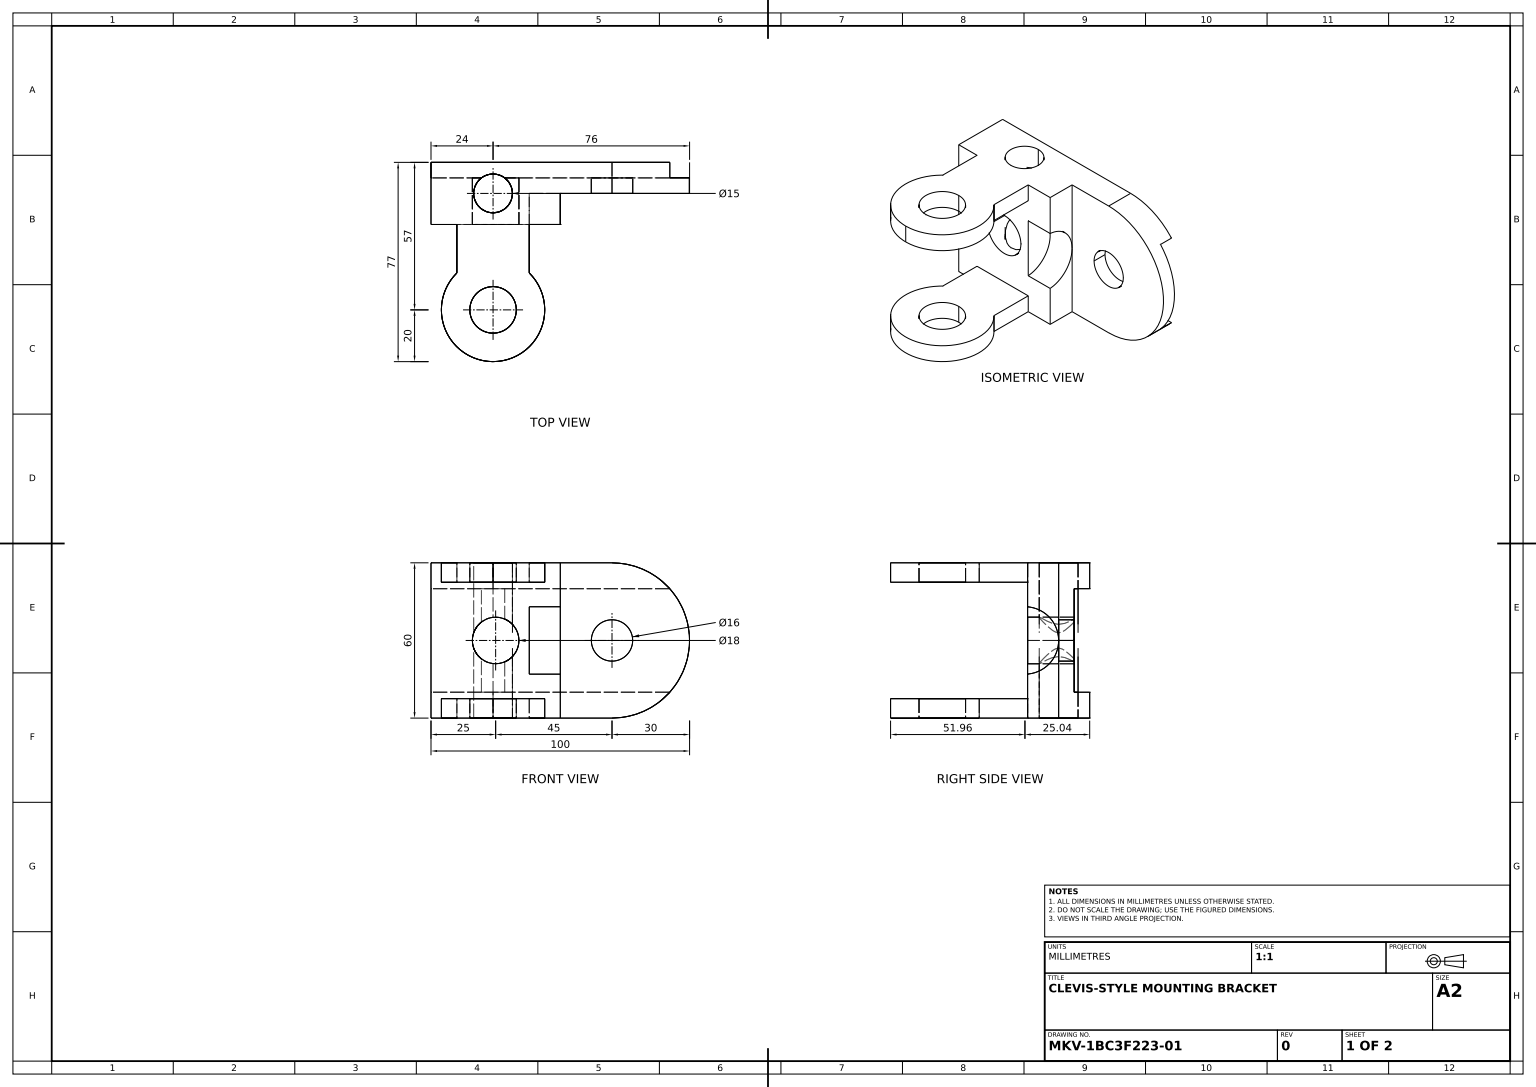
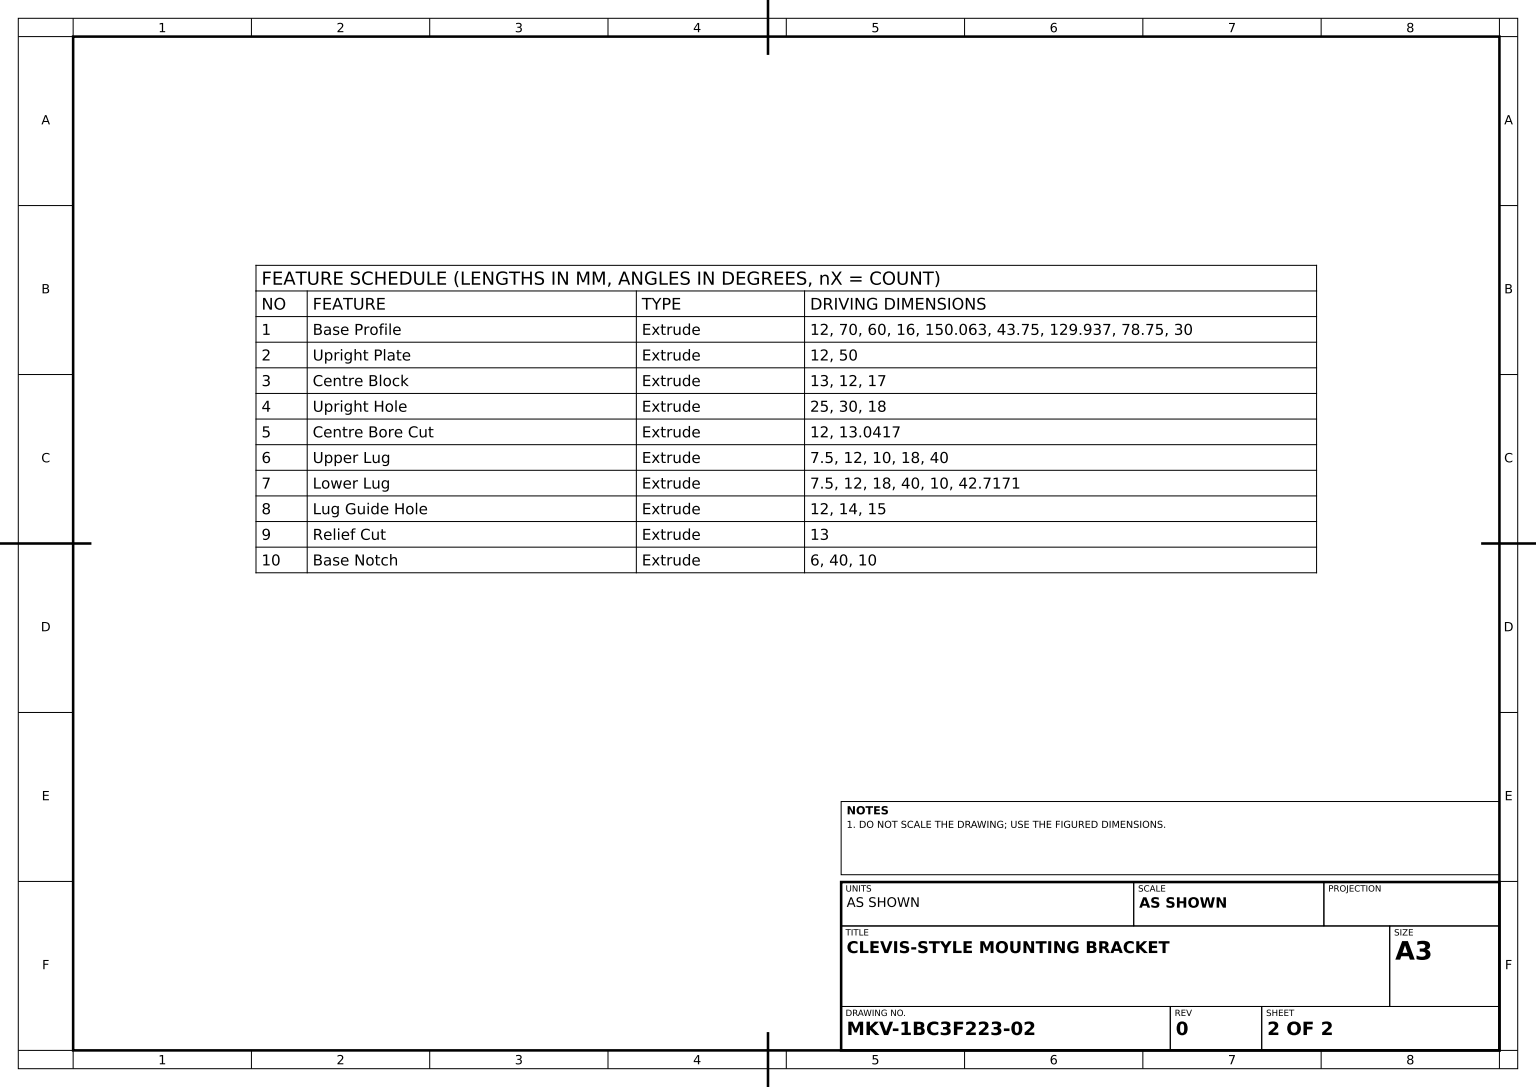
ISO-10303-21;
HEADER;
FILE_DESCRIPTION((''),'2;1');
FILE_NAME('','',(''),(''),'','','');
FILE_SCHEMA(('AUTOMOTIVE_DESIGN'));
ENDSEC;
DATA;
#1=APPLICATION_CONTEXT('');
#2=PRODUCT_CONTEXT('',#1,'mechanical');
#3=PRODUCT('','','',(#2));
#4=PRODUCT_DEFINITION_FORMATION('','',#3);
#5=PRODUCT_DEFINITION_CONTEXT('',#1,'design');
#6=PRODUCT_DEFINITION('','',#4,#5);
#7=PRODUCT_DEFINITION_SHAPE('','',#6);
#8=(LENGTH_UNIT()NAMED_UNIT(*)SI_UNIT(.MILLI.,.METRE.));
#9=(NAMED_UNIT(*)PLANE_ANGLE_UNIT()SI_UNIT($,.RADIAN.));
#10=(NAMED_UNIT(*)SI_UNIT($,.STERADIAN.)SOLID_ANGLE_UNIT());
#11=UNCERTAINTY_MEASURE_WITH_UNIT(LENGTH_MEASURE(1.E-05),#8,'distance_accuracy_value','');
#12=(GEOMETRIC_REPRESENTATION_CONTEXT(3)GLOBAL_UNCERTAINTY_ASSIGNED_CONTEXT((#11))GLOBAL_UNIT_ASSIGNED_CONTEXT((#8,#9,#10))REPRESENTATION_CONTEXT('',''));
#13=CARTESIAN_POINT('',(78.,30.,6.));
#14=VERTEX_POINT('',#13);
#15=CARTESIAN_POINT('',(78.,30.,0.));
#16=VERTEX_POINT('',#15);
#17=DIRECTION('',(0.,0.,-1.));
#18=VECTOR('',#17,1000.);
#19=LINE('',#13,#18);
#20=EDGE_CURVE('',#14,#16,#19,.T.);
#21=ORIENTED_EDGE('',*,*,#20,.F.);
#22=CARTESIAN_POINT('',(62.,30.,6.));
#23=VERTEX_POINT('',#22);
#24=CARTESIAN_POINT('',(70.,30.,6.));
#25=DIRECTION('',(0.,0.,1.));
#26=DIRECTION('',(1.,0.,0.));
#27=AXIS2_PLACEMENT_3D('',#24,#25,#26);
#28=CIRCLE('',#27,8.);
#29=EDGE_CURVE('',#14,#23,#28,.T.);
#30=ORIENTED_EDGE('',*,*,#29,.T.);
#31=CARTESIAN_POINT('',(62.,30.,0.));
#32=VERTEX_POINT('',#31);
#33=LINE('',#22,#18);
#34=EDGE_CURVE('',#23,#32,#33,.T.);
#35=ORIENTED_EDGE('',*,*,#34,.T.);
#36=CARTESIAN_POINT('',(70.,30.,0.));
#37=DIRECTION('',(0.,-1.,0.));
#38=AXIS2_PLACEMENT_3D('',#36,#25,#37);
#39=CIRCLE('',#38,8.);
#40=EDGE_CURVE('',#16,#32,#39,.T.);
#41=ORIENTED_EDGE('',*,*,#40,.F.);
#42=EDGE_LOOP('',(#21,#30,#35,#41));
#43=FACE_OUTER_BOUND('',#42,.T.);
#44=DIRECTION('',(-1.,0.,0.));
#45=AXIS2_PLACEMENT_3D('',#24,#17,#44);
#46=CYLINDRICAL_SURFACE('',#45,8.);
#47=ADVANCED_FACE('',(#43),#46,.F.);
#48=CARTESIAN_POINT('',(24.,52.5,71.));
#49=VERTEX_POINT('',#48);
#50=CARTESIAN_POINT('',(24.,60.,71.));
#51=VERTEX_POINT('',#50);
#52=DIRECTION('',(0.,1.,0.));
#53=VECTOR('',#52,1000.);
#54=LINE('',#48,#53);
#55=EDGE_CURVE('',#49,#51,#54,.T.);
#56=ORIENTED_EDGE('',*,*,#55,.F.);
#57=CARTESIAN_POINT('',(38.,52.5,36.717143));
#58=VERTEX_POINT('',#57);
#59=CARTESIAN_POINT('',(24.,52.5,51.));
#60=AXIS2_PLACEMENT_3D('',#59,#52,#25);
#61=CIRCLE('',#60,20.);
#62=EDGE_CURVE('',#49,#58,#61,.T.);
#63=ORIENTED_EDGE('',*,*,#62,.T.);
#64=CARTESIAN_POINT('',(38.,60.,36.717143));
#65=VERTEX_POINT('',#64);
#66=LINE('',#57,#53);
#67=EDGE_CURVE('',#58,#65,#66,.T.);
#68=ORIENTED_EDGE('',*,*,#67,.T.);
#69=CARTESIAN_POINT('',(24.,60.,51.));
#70=AXIS2_PLACEMENT_3D('',#69,#52,#25);
#71=CIRCLE('',#70,20.);
#72=EDGE_CURVE('',#51,#65,#71,.T.);
#73=ORIENTED_EDGE('',*,*,#72,.F.);
#74=EDGE_LOOP('',(#56,#63,#68,#73));
#75=FACE_OUTER_BOUND('',#74,.T.);
#76=CYLINDRICAL_SURFACE('',#60,20.);
#77=ADVANCED_FACE('',(#75),#76,.T.);
#78=CARTESIAN_POINT('',(24.,7.5,42.));
#79=VERTEX_POINT('',#78);
#80=CARTESIAN_POINT('',(24.,7.5,60.));
#81=VERTEX_POINT('',#80);
#82=CARTESIAN_POINT('',(24.,7.5,51.));
#83=AXIS2_PLACEMENT_3D('',#82,#37,#17);
#84=CIRCLE('',#83,9.);
#85=EDGE_CURVE('',#79,#81,#84,.T.);
#86=ORIENTED_EDGE('',*,*,#85,.F.);
#87=CARTESIAN_POINT('',(24.,0.,42.));
#88=VERTEX_POINT('',#87);
#89=VECTOR('',#37,1000.);
#90=LINE('',#78,#89);
#91=EDGE_CURVE('',#79,#88,#90,.T.);
#92=ORIENTED_EDGE('',*,*,#91,.T.);
#93=CARTESIAN_POINT('',(24.,0.,60.));
#94=VERTEX_POINT('',#93);
#95=CARTESIAN_POINT('',(24.,0.,51.));
#96=AXIS2_PLACEMENT_3D('',#95,#37,#17);
#97=CIRCLE('',#96,9.);
#98=EDGE_CURVE('',#88,#94,#97,.T.);
#99=ORIENTED_EDGE('',*,*,#98,.T.);
#100=LINE('',#80,#89);
#101=EDGE_CURVE('',#81,#94,#100,.T.);
#102=ORIENTED_EDGE('',*,*,#101,.F.);
#103=EDGE_LOOP('',(#86,#92,#99,#102));
#104=FACE_OUTER_BOUND('',#103,.T.);
#105=CYLINDRICAL_SURFACE('',#83,9.);
#106=ADVANCED_FACE('',(#104),#105,.F.);
#107=CARTESIAN_POINT('',(24.,21.055728,13.5));
#108=VERTEX_POINT('',#107);
#109=CARTESIAN_POINT('',(19.5,22.876097,0.));
#110=VERTEX_POINT('',#109);
#111=CARTESIAN_POINT('',(23.775993,21.080773,13.5));
#112=CARTESIAN_POINT('',(23.550071,21.114711,13.489784));
#113=CARTESIAN_POINT('',(23.107751,21.198293,13.450047));
#114=CARTESIAN_POINT('',(22.890357,21.247949,13.420639));
#115=CARTESIAN_POINT('',(22.462687,21.362232,13.343968));
#116=CARTESIAN_POINT('',(22.252411,21.426861,13.2967));
#117=CARTESIAN_POINT('',(21.838724,21.57063,13.185039));
#118=CARTESIAN_POINT('',(21.634861,21.650046,13.120389));
#119=CARTESIAN_POINT('',(21.044654,21.904396,12.905881));
#120=CARTESIAN_POINT('',(20.675526,22.096531,12.734782));
#121=CARTESIAN_POINT('',(20.15335,22.413732,12.441516));
#122=CARTESIAN_POINT('',(19.984095,22.524718,12.337229));
#123=CARTESIAN_POINT('',(19.660446,22.752358,12.12015));
#124=CARTESIAN_POINT('',(19.505485,22.869309,12.007096));
#125=CARTESIAN_POINT('',(19.059315,23.228437,11.65536));
#126=CARTESIAN_POINT('',(18.786705,23.478883,11.404229));
#127=CARTESIAN_POINT('',(18.284964,23.99681,10.870575));
#128=CARTESIAN_POINT('',(18.054749,24.265983,10.586288));
#129=CARTESIAN_POINT('',(17.642159,24.806,9.994734));
#130=CARTESIAN_POINT('',(17.4593,25.077068,9.687637));
#131=CARTESIAN_POINT('',(17.136369,25.611296,9.044665));
#132=CARTESIAN_POINT('',(16.996228,25.87503,8.7093));
#133=CARTESIAN_POINT('',(16.759147,26.371767,7.990771));
#134=CARTESIAN_POINT('',(16.663363,26.6036,7.61237));
#135=CARTESIAN_POINT('',(16.562828,26.865851,6.991193));
#136=CARTESIAN_POINT('',(16.537154,26.936892,6.777549));
#137=CARTESIAN_POINT('',(16.504357,27.029068,6.337619));
#138=CARTESIAN_POINT('',(16.497413,27.049385,6.107487));
#139=CARTESIAN_POINT('',(16.504409,27.029302,5.658707));
#140=CARTESIAN_POINT('',(16.518013,26.989959,5.436381));
#141=CARTESIAN_POINT('',(16.563545,26.864609,5.001537));
#142=CARTESIAN_POINT('',(16.594653,26.781176,4.794949));
#143=CARTESIAN_POINT('',(16.670787,26.589005,4.395648));
#144=CARTESIAN_POINT('',(16.716042,26.479747,4.202338));
#145=CARTESIAN_POINT('',(16.818713,26.247309,3.828192));
#146=CARTESIAN_POINT('',(16.875774,26.124861,3.648443));
#147=CARTESIAN_POINT('',(17.06325,25.747114,3.124382));
#148=CARTESIAN_POINT('',(17.209836,25.481816,2.794887));
#149=CARTESIAN_POINT('',(17.547302,24.944514,2.160499));
#150=CARTESIAN_POINT('',(17.739411,24.670749,1.854583));
#151=CARTESIAN_POINT('',(18.377789,23.866924,0.984166));
#152=CARTESIAN_POINT('',(18.884956,23.350941,0.461283));
#153=B_SPLINE_CURVE_WITH_KNOTS('',3,(#107,#111,#112,#113,#114,#115,#116,#117,#118,#119,#120,#121,#122,#123,#124,#125,#126,#127,#128,#129,#130,#131,#132,#133,#134,#135,#136,#137,#138,#139,#140,#141,#142,#143,#144,#145,#146,#147,#148,#149,#150,#151,#152,#109),.UNSPECIFIED.,.F.,.F.,(4,2,2,2,2,2,2,2,2,2,2,2,2,2,2,2,2,2,2,2,2,4),(0.02427784,0.024948876,0.025619911,0.026290947,0.026961983,0.028304054,0.028975089,0.029646125,0.030988196,0.032330267,0.033672339,0.03501441,0.036356481,0.037027517,0.037698552,0.038369588,0.039040624,0.039711659,0.040382695,0.041724766,0.043066837,0.04575098),.UNSPECIFIED.);
#154=EDGE_CURVE('',#108,#110,#153,.T.);
#155=ORIENTED_EDGE('',*,*,#154,.T.);
#156=CARTESIAN_POINT('',(16.,30.,0.));
#157=VERTEX_POINT('',#156);
#158=CARTESIAN_POINT('',(25.,30.,0.));
#159=AXIS2_PLACEMENT_3D('',#158,#17,#37);
#160=CIRCLE('',#159,9.);
#161=EDGE_CURVE('',#110,#157,#160,.T.);
#162=ORIENTED_EDGE('',*,*,#161,.T.);
#163=CARTESIAN_POINT('',(16.,30.,18.));
#164=VERTEX_POINT('',#163);
#165=CARTESIAN_POINT('',(16.,30.,-6.));
#166=VECTOR('',#25,1000.);
#167=LINE('',#165,#166);
#168=EDGE_CURVE('',#157,#164,#167,.T.);
#169=ORIENTED_EDGE('',*,*,#168,.T.);
#170=CARTESIAN_POINT('',(34.,30.,18.));
#171=VERTEX_POINT('',#170);
#172=CARTESIAN_POINT('',(25.,30.,18.));
#173=AXIS2_PLACEMENT_3D('',#172,#25,#26);
#174=CIRCLE('',#173,9.);
#175=EDGE_CURVE('',#164,#171,#174,.T.);
#176=ORIENTED_EDGE('',*,*,#175,.T.);
#177=CARTESIAN_POINT('',(34.,30.,0.));
#178=VERTEX_POINT('',#177);
#179=CARTESIAN_POINT('',(34.,30.,-6.));
#180=LINE('',#179,#166);
#181=EDGE_CURVE('',#178,#171,#180,.T.);
#182=ORIENTED_EDGE('',*,*,#181,.F.);
#183=CARTESIAN_POINT('',(28.5,21.708438,0.));
#184=VERTEX_POINT('',#183);
#185=EDGE_CURVE('',#178,#184,#160,.T.);
#186=ORIENTED_EDGE('',*,*,#185,.T.);
#187=CARTESIAN_POINT('',(28.80776,21.838348,0.23082));
#188=CARTESIAN_POINT('',(29.093843,21.979213,0.482068));
#189=CARTESIAN_POINT('',(29.626197,22.274013,1.025995));
#190=CARTESIAN_POINT('',(29.870188,22.426886,1.316818));
#191=CARTESIAN_POINT('',(30.309026,22.727791,1.927226));
#192=CARTESIAN_POINT('',(30.505381,22.876742,2.248267));
#193=CARTESIAN_POINT('',(30.85243,23.159014,2.927594));
#194=CARTESIAN_POINT('',(31.002994,23.29242,3.287107));
#195=CARTESIAN_POINT('',(31.246347,23.518432,4.02714));
#196=CARTESIAN_POINT('',(31.340739,23.612247,4.410234));
#197=CARTESIAN_POINT('',(31.469188,23.742368,5.209415));
#198=CARTESIAN_POINT('',(31.500892,23.775982,5.613918));
#199=CARTESIAN_POINT('',(31.499525,23.774554,6.218485));
#200=CARTESIAN_POINT('',(31.49096,23.765578,6.420154));
#201=CARTESIAN_POINT('',(31.457371,23.730794,6.823786));
#202=CARTESIAN_POINT('',(31.432094,23.704734,7.026948));
#203=CARTESIAN_POINT('',(31.333251,23.60479,7.623568));
#204=CARTESIAN_POINT('',(31.237132,23.509482,8.006825));
#205=CARTESIAN_POINT('',(31.050818,23.337061,8.564043));
#206=CARTESIAN_POINT('',(30.981359,23.27443,8.747342));
#207=CARTESIAN_POINT('',(30.830785,23.143477,9.102844));
#208=CARTESIAN_POINT('',(30.749491,23.074979,9.275724));
#209=CARTESIAN_POINT('',(30.488091,22.863396,9.781359));
#210=CARTESIAN_POINT('',(30.290618,22.714318,10.101238));
#211=CARTESIAN_POINT('',(29.847811,22.412476,10.71117));
#212=CARTESIAN_POINT('',(29.600622,22.258788,11.002619));
#213=CARTESIAN_POINT('',(29.068708,21.966464,11.540881));
#214=CARTESIAN_POINT('',(28.782935,21.826843,11.789674));
#215=CARTESIAN_POINT('',(28.321771,21.633782,12.132617));
#216=CARTESIAN_POINT('',(28.162605,21.572155,12.241856));
#217=CARTESIAN_POINT('',(27.832514,21.455557,12.449797));
#218=CARTESIAN_POINT('',(27.660707,21.400356,12.548922));
#219=CARTESIAN_POINT('',(27.135088,21.249324,12.824796));
#220=CARTESIAN_POINT('',(26.770139,21.167389,12.98123));
#221=CARTESIAN_POINT('',(26.008904,21.048435,13.237095));
#222=CARTESIAN_POINT('',(25.608077,21.011639,13.336802));
#223=CARTESIAN_POINT('',(24.807296,20.993155,13.467453));
#224=CARTESIAN_POINT('',(24.404712,21.01048,13.5));
#225=B_SPLINE_CURVE_WITH_KNOTS('',3,(#183,#187,#188,#189,#190,#191,#192,#193,#194,#195,#196,#197,#198,#199,#200,#201,#202,#203,#204,#205,#206,#207,#208,#209,#210,#211,#212,#213,#214,#215,#216,#217,#218,#219,#220,#221,#222,#223,#224,#107),.UNSPECIFIED.,.F.,.F.,(4,2,2,2,2,2,2,2,2,2,2,2,2,2,2,2,2,2,2,4),(0.004880127,0.006092484,0.007304841,0.008517198,0.009729555,0.010941912,0.012154269,0.012760448,0.013366627,0.014578984,0.015185162,0.015791341,0.017003698,0.018216055,0.019428412,0.02003459,0.020640769,0.021853126,0.023065483,0.02427784),.UNSPECIFIED.);
#226=EDGE_CURVE('',#184,#108,#225,.T.);
#227=ORIENTED_EDGE('',*,*,#226,.T.);
#228=EDGE_LOOP('',(#155,#162,#169,#176,#182,#186,#227));
#229=FACE_OUTER_BOUND('',#228,.T.);
#230=CARTESIAN_POINT('',(25.,30.,-6.));
#231=AXIS2_PLACEMENT_3D('',#230,#25,#26);
#232=CYLINDRICAL_SURFACE('',#231,9.);
#233=ADVANCED_FACE('',(#229),#232,.F.);
#234=CARTESIAN_POINT('',(28.5,10.,0.));
#235=VERTEX_POINT('',#234);
#236=CARTESIAN_POINT('',(24.,10.,-1.5));
#237=VERTEX_POINT('',#236);
#238=CARTESIAN_POINT('',(24.,10.,6.));
#239=AXIS2_PLACEMENT_3D('',#238,#52,#17);
#240=CIRCLE('',#239,7.5);
#241=EDGE_CURVE('',#235,#237,#240,.T.);
#242=ORIENTED_EDGE('',*,*,#241,.T.);
#243=CARTESIAN_POINT('',(24.,0.,-1.5));
#244=VERTEX_POINT('',#243);
#245=CARTESIAN_POINT('',(24.,60.,-1.5));
#246=LINE('',#245,#89);
#247=EDGE_CURVE('',#237,#244,#246,.T.);
#248=ORIENTED_EDGE('',*,*,#247,.T.);
#249=CARTESIAN_POINT('',(24.,0.,13.5));
#250=VERTEX_POINT('',#249);
#251=CARTESIAN_POINT('',(24.,0.,6.));
#252=AXIS2_PLACEMENT_3D('',#251,#37,#17);
#253=CIRCLE('',#252,7.5);
#254=EDGE_CURVE('',#244,#250,#253,.T.);
#255=ORIENTED_EDGE('',*,*,#254,.T.);
#256=CARTESIAN_POINT('',(24.,60.,13.5));
#257=LINE('',#256,#89);
#258=EDGE_CURVE('',#108,#250,#257,.T.);
#259=ORIENTED_EDGE('',*,*,#258,.F.);
#260=ORIENTED_EDGE('',*,*,#226,.F.);
#261=CARTESIAN_POINT('',(28.5,60.,0.));
#262=LINE('',#261,#89);
#263=EDGE_CURVE('',#184,#235,#262,.T.);
#264=ORIENTED_EDGE('',*,*,#263,.T.);
#265=EDGE_LOOP('',(#242,#248,#255,#259,#260,#264));
#266=FACE_OUTER_BOUND('',#265,.T.);
#267=CARTESIAN_POINT('',(24.,60.,6.));
#268=AXIS2_PLACEMENT_3D('',#267,#37,#17);
#269=CYLINDRICAL_SURFACE('',#268,7.5);
#270=ADVANCED_FACE('',(#266),#269,.F.);
#271=CARTESIAN_POINT('',(0.,0.,-6.));
#272=VERTEX_POINT('',#271);
#273=CARTESIAN_POINT('',(70.,0.,-6.));
#274=VERTEX_POINT('',#273);
#275=VECTOR('',#26,1000.);
#276=LINE('',#271,#275);
#277=EDGE_CURVE('',#272,#274,#276,.T.);
#278=ORIENTED_EDGE('',*,*,#277,.F.);
#279=CARTESIAN_POINT('',(0.,10.,-6.));
#280=VERTEX_POINT('',#279);
#281=LINE('',#271,#89);
#282=EDGE_CURVE('',#280,#272,#281,.T.);
#283=ORIENTED_EDGE('',*,*,#282,.F.);
#284=CARTESIAN_POINT('',(92.36068,10.,-6.));
#285=VERTEX_POINT('',#284);
#286=CARTESIAN_POINT('',(100.,10.,-6.));
#287=VECTOR('',#44,1000.);
#288=LINE('',#286,#287);
#289=EDGE_CURVE('',#285,#280,#288,.T.);
#290=ORIENTED_EDGE('',*,*,#289,.F.);
#291=CARTESIAN_POINT('',(70.,30.,-6.));
#292=AXIS2_PLACEMENT_3D('',#291,#25,#44);
#293=CIRCLE('',#292,30.);
#294=EDGE_CURVE('',#274,#285,#293,.T.);
#295=ORIENTED_EDGE('',*,*,#294,.F.);
#296=EDGE_LOOP('',(#278,#283,#290,#295));
#297=FACE_OUTER_BOUND('',#296,.T.);
#298=AXIS2_PLACEMENT_3D('',#291,#17,#44);
#299=PLANE('',#298);
#300=ADVANCED_FACE('',(#297),#299,.T.);
#301=VERTEX_POINT('',#256);
#302=VERTEX_POINT('',#245);
#303=CIRCLE('',#268,7.5);
#304=EDGE_CURVE('',#301,#302,#303,.T.);
#305=ORIENTED_EDGE('',*,*,#304,.F.);
#306=CARTESIAN_POINT('',(24.,38.944272,13.5));
#307=VERTEX_POINT('',#306);
#308=EDGE_CURVE('',#301,#307,#257,.T.);
#309=ORIENTED_EDGE('',*,*,#308,.T.);
#310=CARTESIAN_POINT('',(19.5,37.123903,0.));
#311=VERTEX_POINT('',#310);
#312=CARTESIAN_POINT('',(19.194209,36.887818,0.229343));
#313=CARTESIAN_POINT('',(18.914049,36.640294,0.475662));
#314=CARTESIAN_POINT('',(18.398038,36.127511,0.999677));
#315=CARTESIAN_POINT('',(18.161311,35.860973,1.27866));
#316=CARTESIAN_POINT('',(17.733291,35.321055,1.863612));
#317=CARTESIAN_POINT('',(17.543306,35.049569,2.167234));
#318=CARTESIAN_POINT('',(17.206612,34.512596,2.80174));
#319=CARTESIAN_POINT('',(17.059862,34.246648,3.132225));
#320=CARTESIAN_POINT('',(16.809169,33.740332,3.836302));
#321=CARTESIAN_POINT('',(16.705325,33.498712,4.209522));
#322=CARTESIAN_POINT('',(16.591547,33.210697,4.813894));
#323=CARTESIAN_POINT('',(16.560467,33.127049,5.025057));
#324=CARTESIAN_POINT('',(16.516515,33.005767,5.457212));
#325=CARTESIAN_POINT('',(16.503296,32.967505,5.682374));
#326=CARTESIAN_POINT('',(16.497803,32.951732,6.136051));
#327=CARTESIAN_POINT('',(16.505357,32.973826,6.359448));
#328=CARTESIAN_POINT('',(16.53954,33.069725,6.800255));
#329=CARTESIAN_POINT('',(16.566196,33.143211,7.015632));
#330=CARTESIAN_POINT('',(16.667338,33.406174,7.629067));
#331=CARTESIAN_POINT('',(16.764521,33.640344,8.009695));
#332=CARTESIAN_POINT('',(17.001475,34.135072,8.722441));
#333=CARTESIAN_POINT('',(17.141747,34.398374,9.056791));
#334=CARTESIAN_POINT('',(17.466063,34.933318,9.699631));
#335=CARTESIAN_POINT('',(17.651258,35.206871,10.009157));
#336=CARTESIAN_POINT('',(18.271703,36.015985,10.894494));
#337=CARTESIAN_POINT('',(18.766256,36.536834,11.425685));
#338=CARTESIAN_POINT('',(19.664473,37.258071,12.13174));
#339=CARTESIAN_POINT('',(19.989971,37.487517,12.35032));
#340=CARTESIAN_POINT('',(20.681179,37.906396,12.737383));
#341=CARTESIAN_POINT('',(21.049,38.09777,12.907789));
#342=CARTESIAN_POINT('',(21.640505,38.352237,13.122273));
#343=CARTESIAN_POINT('',(21.843639,38.431184,13.186484));
#344=CARTESIAN_POINT('',(22.255334,38.574047,13.297369));
#345=CARTESIAN_POINT('',(22.464845,38.638388,13.344404));
#346=CARTESIAN_POINT('',(22.891523,38.752319,13.420799));
#347=CARTESIAN_POINT('',(23.108689,38.801911,13.450162));
#348=CARTESIAN_POINT('',(23.551192,38.885474,13.489854));
#349=CARTESIAN_POINT('',(23.776558,38.91929,13.5));
#350=B_SPLINE_CURVE_WITH_KNOTS('',3,(#310,#312,#313,#314,#315,#316,#317,#318,#319,#320,#321,#322,#323,#324,#325,#326,#327,#328,#329,#330,#331,#332,#333,#334,#335,#336,#337,#338,#339,#340,#341,#342,#343,#344,#345,#346,#347,#348,#349,#306),.UNSPECIFIED.,.F.,.F.,(4,2,2,2,2,2,2,2,2,2,2,2,2,2,2,2,2,2,2,4),(0.005166857,0.006510904,0.007854951,0.009198998,0.010543046,0.011887093,0.012559117,0.01323114,0.013903164,0.014575187,0.015919235,0.017263282,0.018607329,0.021295423,0.022639471,0.023983518,0.024655542,0.025327565,0.025999589,0.026671612),.UNSPECIFIED.);
#351=EDGE_CURVE('',#311,#307,#350,.T.);
#352=ORIENTED_EDGE('',*,*,#351,.F.);
#353=CARTESIAN_POINT('',(19.5,50.,0.));
#354=VERTEX_POINT('',#353);
#355=CARTESIAN_POINT('',(19.5,60.,0.));
#356=LINE('',#355,#53);
#357=EDGE_CURVE('',#311,#354,#356,.T.);
#358=ORIENTED_EDGE('',*,*,#357,.T.);
#359=CARTESIAN_POINT('',(24.,50.,-1.5));
#360=VERTEX_POINT('',#359);
#361=CARTESIAN_POINT('',(24.,50.,6.));
#362=AXIS2_PLACEMENT_3D('',#361,#37,#25);
#363=CIRCLE('',#362,7.5);
#364=EDGE_CURVE('',#354,#360,#363,.T.);
#365=ORIENTED_EDGE('',*,*,#364,.T.);
#366=EDGE_CURVE('',#302,#360,#246,.T.);
#367=ORIENTED_EDGE('',*,*,#366,.F.);
#368=EDGE_LOOP('',(#305,#309,#352,#358,#365,#367));
#369=FACE_OUTER_BOUND('',#368,.T.);
#370=ADVANCED_FACE('',(#369),#269,.F.);
#371=CARTESIAN_POINT('',(10.,52.5,36.717143));
#372=VERTEX_POINT('',#371);
#373=EDGE_CURVE('',#372,#49,#61,.T.);
#374=ORIENTED_EDGE('',*,*,#373,.F.);
#375=CARTESIAN_POINT('',(10.,52.5,18.));
#376=VERTEX_POINT('',#375);
#377=CARTESIAN_POINT('',(10.,52.5,6.));
#378=LINE('',#377,#166);
#379=EDGE_CURVE('',#376,#372,#378,.T.);
#380=ORIENTED_EDGE('',*,*,#379,.F.);
#381=CARTESIAN_POINT('',(38.,52.5,18.));
#382=VERTEX_POINT('',#381);
#383=CARTESIAN_POINT('',(0.,52.5,18.));
#384=LINE('',#383,#287);
#385=EDGE_CURVE('',#382,#376,#384,.T.);
#386=ORIENTED_EDGE('',*,*,#385,.F.);
#387=LINE('',#57,#18);
#388=EDGE_CURVE('',#58,#382,#387,.T.);
#389=ORIENTED_EDGE('',*,*,#388,.F.);
#390=ORIENTED_EDGE('',*,*,#62,.F.);
#391=EDGE_LOOP('',(#374,#380,#386,#389,#390));
#392=FACE_OUTER_BOUND('',#391,.T.);
#393=CARTESIAN_POINT('',(24.,52.5,42.));
#394=VERTEX_POINT('',#393);
#395=CARTESIAN_POINT('',(24.,52.5,60.));
#396=VERTEX_POINT('',#395);
#397=CIRCLE('',#60,9.);
#398=EDGE_CURVE('',#394,#396,#397,.T.);
#399=ORIENTED_EDGE('',*,*,#398,.T.);
#400=EDGE_CURVE('',#396,#394,#397,.T.);
#401=ORIENTED_EDGE('',*,*,#400,.T.);
#402=EDGE_LOOP('',(#399,#401));
#403=FACE_BOUND('',#402,.T.);
#404=PLANE('',#60);
#405=ADVANCED_FACE('',(#392,#403),#404,.F.);
#406=CARTESIAN_POINT('',(19.5,10.,0.));
#407=VERTEX_POINT('',#406);
#408=EDGE_CURVE('',#407,#110,#356,.T.);
#409=ORIENTED_EDGE('',*,*,#408,.T.);
#410=ORIENTED_EDGE('',*,*,#154,.F.);
#411=ORIENTED_EDGE('',*,*,#258,.T.);
#412=EDGE_CURVE('',#250,#244,#253,.T.);
#413=ORIENTED_EDGE('',*,*,#412,.T.);
#414=ORIENTED_EDGE('',*,*,#247,.F.);
#415=EDGE_CURVE('',#237,#407,#240,.T.);
#416=ORIENTED_EDGE('',*,*,#415,.T.);
#417=EDGE_LOOP('',(#409,#410,#411,#413,#414,#416));
#418=FACE_OUTER_BOUND('',#417,.T.);
#419=ADVANCED_FACE('',(#418),#269,.F.);
#420=ORIENTED_EDGE('',*,*,#379,.T.);
#421=CARTESIAN_POINT('',(10.,60.,36.717143));
#422=VERTEX_POINT('',#421);
#423=LINE('',#371,#53);
#424=EDGE_CURVE('',#372,#422,#423,.T.);
#425=ORIENTED_EDGE('',*,*,#424,.T.);
#426=CARTESIAN_POINT('',(10.,60.,18.));
#427=VERTEX_POINT('',#426);
#428=CARTESIAN_POINT('',(10.,60.,6.));
#429=LINE('',#428,#166);
#430=EDGE_CURVE('',#427,#422,#429,.T.);
#431=ORIENTED_EDGE('',*,*,#430,.F.);
#432=CARTESIAN_POINT('',(10.,0.,18.));
#433=LINE('',#432,#89);
#434=EDGE_CURVE('',#427,#376,#433,.T.);
#435=ORIENTED_EDGE('',*,*,#434,.T.);
#436=EDGE_LOOP('',(#420,#425,#431,#435));
#437=FACE_OUTER_BOUND('',#436,.T.);
#438=AXIS2_PLACEMENT_3D('',#377,#44,#25);
#439=PLANE('',#438);
#440=ADVANCED_FACE('',(#437),#439,.T.);
#441=CARTESIAN_POINT('',(0.,10.,0.));
#442=VERTEX_POINT('',#441);
#443=CARTESIAN_POINT('',(100.,10.,0.));
#444=LINE('',#443,#287);
#445=EDGE_CURVE('',#407,#442,#444,.T.);
#446=ORIENTED_EDGE('',*,*,#445,.T.);
#447=CARTESIAN_POINT('',(0.,50.,0.));
#448=VERTEX_POINT('',#447);
#449=LINE('',#447,#53);
#450=EDGE_CURVE('',#442,#448,#449,.T.);
#451=ORIENTED_EDGE('',*,*,#450,.T.);
#452=CARTESIAN_POINT('',(100.,50.,0.));
#453=LINE('',#452,#287);
#454=EDGE_CURVE('',#354,#448,#453,.T.);
#455=ORIENTED_EDGE('',*,*,#454,.F.);
#456=ORIENTED_EDGE('',*,*,#357,.F.);
#457=EDGE_CURVE('',#157,#311,#160,.T.);
#458=ORIENTED_EDGE('',*,*,#457,.F.);
#459=ORIENTED_EDGE('',*,*,#161,.F.);
#460=ORIENTED_EDGE('',*,*,#408,.F.);
#461=EDGE_LOOP('',(#446,#451,#455,#456,#458,#459,#460));
#462=FACE_OUTER_BOUND('',#461,.T.);
#463=AXIS2_PLACEMENT_3D('',#452,#25,#37);
#464=PLANE('',#463);
#465=ADVANCED_FACE('',(#462),#464,.F.);
#466=CARTESIAN_POINT('',(92.36068,50.,0.));
#467=VERTEX_POINT('',#466);
#468=CARTESIAN_POINT('',(28.5,50.,0.));
#469=VERTEX_POINT('',#468);
#470=EDGE_CURVE('',#467,#469,#453,.T.);
#471=ORIENTED_EDGE('',*,*,#470,.F.);
#472=CARTESIAN_POINT('',(92.36068,10.,0.));
#473=VERTEX_POINT('',#472);
#474=CIRCLE('',#38,30.);
#475=EDGE_CURVE('',#473,#467,#474,.T.);
#476=ORIENTED_EDGE('',*,*,#475,.F.);
#477=EDGE_CURVE('',#473,#235,#444,.T.);
#478=ORIENTED_EDGE('',*,*,#477,.T.);
#479=ORIENTED_EDGE('',*,*,#263,.F.);
#480=ORIENTED_EDGE('',*,*,#185,.F.);
#481=CARTESIAN_POINT('',(28.5,38.291562,0.));
#482=VERTEX_POINT('',#481);
#483=EDGE_CURVE('',#482,#178,#160,.T.);
#484=ORIENTED_EDGE('',*,*,#483,.F.);
#485=EDGE_CURVE('',#469,#482,#262,.T.);
#486=ORIENTED_EDGE('',*,*,#485,.F.);
#487=EDGE_LOOP('',(#471,#476,#478,#479,#480,#484,#486));
#488=FACE_OUTER_BOUND('',#487,.T.);
#489=EDGE_CURVE('',#32,#16,#39,.T.);
#490=ORIENTED_EDGE('',*,*,#489,.T.);
#491=ORIENTED_EDGE('',*,*,#40,.T.);
#492=EDGE_LOOP('',(#490,#491));
#493=FACE_BOUND('',#492,.T.);
#494=ADVANCED_FACE('',(#488,#493),#464,.F.);
#495=CARTESIAN_POINT('',(24.403234,38.989355,13.5));
#496=CARTESIAN_POINT('',(24.805141,39.006803,13.46769));
#497=CARTESIAN_POINT('',(25.405866,38.993075,13.369851));
#498=CARTESIAN_POINT('',(25.606888,38.981704,13.328664));
#499=CARTESIAN_POINT('',(26.001912,38.946256,13.230751));
#500=CARTESIAN_POINT('',(26.19559,38.922307,13.17423));
#501=CARTESIAN_POINT('',(26.765758,38.833464,12.982931));
#502=CARTESIAN_POINT('',(27.132105,38.751444,12.826224));
#503=CARTESIAN_POINT('',(27.834838,38.549698,12.457665));
#504=CARTESIAN_POINT('',(28.163415,38.432365,12.250108));
#505=CARTESIAN_POINT('',(28.78083,38.174184,11.791506));
#506=CARTESIAN_POINT('',(29.071392,38.032211,11.538512));
#507=CARTESIAN_POINT('',(29.60476,37.738787,10.99808));
#508=CARTESIAN_POINT('',(29.847615,37.58763,10.711346));
#509=CARTESIAN_POINT('',(30.289524,37.286456,10.102839));
#510=CARTESIAN_POINT('',(30.48968,37.13542,9.778879));
#511=CARTESIAN_POINT('',(30.839991,36.851665,9.100064));
#512=CARTESIAN_POINT('',(30.989413,36.719756,8.74755));
#513=CARTESIAN_POINT('',(31.17427,36.548698,8.194901));
#514=CARTESIAN_POINT('',(31.229297,36.49618,8.006676));
#515=CARTESIAN_POINT('',(31.325405,36.402637,7.621088));
#516=CARTESIAN_POINT('',(31.366397,36.361695,7.42354));
#517=CARTESIAN_POINT('',(31.464771,36.262223,6.829622));
#518=CARTESIAN_POINT('',(31.498934,36.226063,6.427687));
#519=CARTESIAN_POINT('',(31.500496,36.224432,5.814831));
#520=CARTESIAN_POINT('',(31.492543,36.23277,5.608966));
#521=CARTESIAN_POINT('',(31.460475,36.266003,5.204753));
#522=CARTESIAN_POINT('',(31.436399,36.290852,5.005008));
#523=CARTESIAN_POINT('',(31.340949,36.387533,4.412352));
#524=CARTESIAN_POINT('',(31.245076,36.482812,4.0223));
#525=CARTESIAN_POINT('',(31.000575,36.709763,3.280741));
#526=CARTESIAN_POINT('',(30.852544,36.840852,2.928061));
#527=CARTESIAN_POINT('',(30.507256,37.121774,2.251694));
#528=CARTESIAN_POINT('',(30.308302,37.272789,1.925938));
#529=CARTESIAN_POINT('',(29.867101,37.575147,1.312807));
#530=CARTESIAN_POINT('',(29.625406,37.726365,1.025328));
#531=CARTESIAN_POINT('',(29.097367,38.018895,0.485528));
#532=CARTESIAN_POINT('',(28.808782,38.16122,0.231586));
#533=B_SPLINE_CURVE_WITH_KNOTS('',3,(#306,#495,#496,#497,#498,#499,#500,#501,#502,#503,#504,#505,#506,#507,#508,#509,#510,#511,#512,#513,#514,#515,#516,#517,#518,#519,#520,#521,#522,#523,#524,#525,#526,#527,#528,#529,#530,#531,#532,#481),.UNSPECIFIED.,.F.,.F.,(4,2,2,2,2,2,2,2,2,2,2,2,2,2,2,2,2,2,2,4),(0.026671612,0.027884378,0.028490761,0.029097144,0.03030991,0.031522676,0.032735443,0.033948209,0.035160975,0.036373741,0.036980124,0.037586507,0.038799273,0.039405656,0.040012039,0.041224805,0.042437571,0.043650337,0.044863103,0.046075869),.UNSPECIFIED.);
#534=EDGE_CURVE('',#307,#482,#533,.T.);
#535=ORIENTED_EDGE('',*,*,#534,.T.);
#536=ORIENTED_EDGE('',*,*,#483,.T.);
#537=ORIENTED_EDGE('',*,*,#181,.T.);
#538=EDGE_CURVE('',#171,#164,#174,.T.);
#539=ORIENTED_EDGE('',*,*,#538,.T.);
#540=ORIENTED_EDGE('',*,*,#168,.F.);
#541=ORIENTED_EDGE('',*,*,#457,.T.);
#542=ORIENTED_EDGE('',*,*,#351,.T.);
#543=EDGE_LOOP('',(#535,#536,#537,#539,#540,#541,#542));
#544=FACE_OUTER_BOUND('',#543,.T.);
#545=ADVANCED_FACE('',(#544),#232,.F.);
#546=EDGE_CURVE('',#94,#88,#97,.T.);
#547=ORIENTED_EDGE('',*,*,#546,.F.);
#548=ORIENTED_EDGE('',*,*,#98,.F.);
#549=EDGE_LOOP('',(#547,#548));
#550=FACE_BOUND('',#549,.T.);
#551=CARTESIAN_POINT('',(38.,0.,18.));
#552=VERTEX_POINT('',#551);
#553=CARTESIAN_POINT('',(50.,0.,18.));
#554=VERTEX_POINT('',#553);
#555=LINE('',#551,#275);
#556=EDGE_CURVE('',#552,#554,#555,.T.);
#557=ORIENTED_EDGE('',*,*,#556,.F.);
#558=CARTESIAN_POINT('',(38.,0.,36.717143));
#559=VERTEX_POINT('',#558);
#560=CARTESIAN_POINT('',(38.,0.,0.));
#561=LINE('',#560,#18);
#562=EDGE_CURVE('',#559,#552,#561,.T.);
#563=ORIENTED_EDGE('',*,*,#562,.F.);
#564=CARTESIAN_POINT('',(10.,0.,36.717143));
#565=VERTEX_POINT('',#564);
#566=CIRCLE('',#96,20.);
#567=EDGE_CURVE('',#559,#565,#566,.T.);
#568=ORIENTED_EDGE('',*,*,#567,.T.);
#569=VERTEX_POINT('',#432);
#570=CARTESIAN_POINT('',(10.,0.,0.));
#571=LINE('',#570,#166);
#572=EDGE_CURVE('',#569,#565,#571,.T.);
#573=ORIENTED_EDGE('',*,*,#572,.F.);
#574=CARTESIAN_POINT('',(0.,0.,18.));
#575=VERTEX_POINT('',#574);
#576=LINE('',#574,#275);
#577=EDGE_CURVE('',#575,#569,#576,.T.);
#578=ORIENTED_EDGE('',*,*,#577,.F.);
#579=CARTESIAN_POINT('',(0.,0.,6.));
#580=LINE('',#579,#18);
#581=EDGE_CURVE('',#575,#272,#580,.T.);
#582=ORIENTED_EDGE('',*,*,#581,.T.);
#583=ORIENTED_EDGE('',*,*,#277,.T.);
#584=CARTESIAN_POINT('',(70.,0.,6.));
#585=VERTEX_POINT('',#584);
#586=LINE('',#584,#18);
#587=EDGE_CURVE('',#585,#274,#586,.T.);
#588=ORIENTED_EDGE('',*,*,#587,.F.);
#589=CARTESIAN_POINT('',(50.,0.,6.));
#590=VERTEX_POINT('',#589);
#591=LINE('',#579,#275);
#592=EDGE_CURVE('',#590,#585,#591,.T.);
#593=ORIENTED_EDGE('',*,*,#592,.F.);
#594=LINE('',#553,#18);
#595=EDGE_CURVE('',#554,#590,#594,.T.);
#596=ORIENTED_EDGE('',*,*,#595,.F.);
#597=EDGE_LOOP('',(#557,#563,#568,#573,#578,#582,#583,#588,#593,#596));
#598=FACE_OUTER_BOUND('',#597,.T.);
#599=ORIENTED_EDGE('',*,*,#412,.F.);
#600=ORIENTED_EDGE('',*,*,#254,.F.);
#601=EDGE_LOOP('',(#599,#600));
#602=FACE_BOUND('',#601,.T.);
#603=AXIS2_PLACEMENT_3D('',#579,#52,#25);
#604=PLANE('',#603);
#605=ADVANCED_FACE('',(#550,#598,#602),#604,.F.);
#606=CARTESIAN_POINT('',(92.36068,50.,-6.));
#607=VERTEX_POINT('',#606);
#608=CARTESIAN_POINT('',(70.,60.,-6.));
#609=VERTEX_POINT('',#608);
#610=EDGE_CURVE('',#607,#609,#293,.T.);
#611=ORIENTED_EDGE('',*,*,#610,.F.);
#612=CARTESIAN_POINT('',(0.,50.,-6.));
#613=VERTEX_POINT('',#612);
#614=CARTESIAN_POINT('',(100.,50.,-6.));
#615=LINE('',#614,#287);
#616=EDGE_CURVE('',#607,#613,#615,.T.);
#617=ORIENTED_EDGE('',*,*,#616,.T.);
#618=CARTESIAN_POINT('',(0.,60.,-6.));
#619=VERTEX_POINT('',#618);
#620=EDGE_CURVE('',#619,#613,#281,.T.);
#621=ORIENTED_EDGE('',*,*,#620,.F.);
#622=LINE('',#618,#287);
#623=EDGE_CURVE('',#609,#619,#622,.T.);
#624=ORIENTED_EDGE('',*,*,#623,.F.);
#625=EDGE_LOOP('',(#611,#617,#621,#624));
#626=FACE_OUTER_BOUND('',#625,.T.);
#627=ADVANCED_FACE('',(#626),#299,.T.);
#628=EDGE_CURVE('',#360,#469,#363,.T.);
#629=ORIENTED_EDGE('',*,*,#628,.T.);
#630=ORIENTED_EDGE('',*,*,#485,.T.);
#631=ORIENTED_EDGE('',*,*,#534,.F.);
#632=ORIENTED_EDGE('',*,*,#308,.F.);
#633=EDGE_CURVE('',#302,#301,#303,.T.);
#634=ORIENTED_EDGE('',*,*,#633,.F.);
#635=ORIENTED_EDGE('',*,*,#366,.T.);
#636=EDGE_LOOP('',(#629,#630,#631,#632,#634,#635));
#637=FACE_OUTER_BOUND('',#636,.T.);
#638=ADVANCED_FACE('',(#637),#269,.F.);
#639=ORIENTED_EDGE('',*,*,#34,.F.);
#640=EDGE_CURVE('',#23,#14,#28,.T.);
#641=ORIENTED_EDGE('',*,*,#640,.T.);
#642=ORIENTED_EDGE('',*,*,#20,.T.);
#643=ORIENTED_EDGE('',*,*,#489,.F.);
#644=EDGE_LOOP('',(#639,#641,#642,#643));
#645=FACE_OUTER_BOUND('',#644,.T.);
#646=ADVANCED_FACE('',(#645),#46,.F.);
#647=ORIENTED_EDGE('',*,*,#289,.T.);
#648=LINE('',#441,#166);
#649=EDGE_CURVE('',#280,#442,#648,.T.);
#650=ORIENTED_EDGE('',*,*,#649,.T.);
#651=ORIENTED_EDGE('',*,*,#445,.F.);
#652=ORIENTED_EDGE('',*,*,#415,.F.);
#653=ORIENTED_EDGE('',*,*,#241,.F.);
#654=ORIENTED_EDGE('',*,*,#477,.F.);
#655=CARTESIAN_POINT('',(92.36068,10.,6.));
#656=LINE('',#655,#166);
#657=EDGE_CURVE('',#285,#473,#656,.T.);
#658=ORIENTED_EDGE('',*,*,#657,.F.);
#659=EDGE_LOOP('',(#647,#650,#651,#652,#653,#654,#658));
#660=FACE_OUTER_BOUND('',#659,.T.);
#661=AXIS2_PLACEMENT_3D('',#443,#37,#17);
#662=PLANE('',#661);
#663=ADVANCED_FACE('',(#660),#662,.F.);
#664=ORIENTED_EDGE('',*,*,#67,.F.);
#665=ORIENTED_EDGE('',*,*,#388,.T.);
#666=CARTESIAN_POINT('',(38.,60.,18.));
#667=VERTEX_POINT('',#666);
#668=LINE('',#666,#89);
#669=EDGE_CURVE('',#667,#382,#668,.T.);
#670=ORIENTED_EDGE('',*,*,#669,.F.);
#671=LINE('',#64,#18);
#672=EDGE_CURVE('',#65,#667,#671,.T.);
#673=ORIENTED_EDGE('',*,*,#672,.F.);
#674=EDGE_LOOP('',(#664,#665,#670,#673));
#675=FACE_OUTER_BOUND('',#674,.T.);
#676=AXIS2_PLACEMENT_3D('',#57,#26,#17);
#677=PLANE('',#676);
#678=ADVANCED_FACE('',(#675),#677,.T.);
#679=ORIENTED_EDGE('',*,*,#101,.T.);
#680=ORIENTED_EDGE('',*,*,#546,.T.);
#681=ORIENTED_EDGE('',*,*,#91,.F.);
#682=EDGE_CURVE('',#81,#79,#84,.T.);
#683=ORIENTED_EDGE('',*,*,#682,.F.);
#684=EDGE_LOOP('',(#679,#680,#681,#683));
#685=FACE_OUTER_BOUND('',#684,.T.);
#686=ADVANCED_FACE('',(#685),#105,.F.);
#687=CARTESIAN_POINT('',(92.36068,50.,6.));
#688=LINE('',#687,#18);
#689=EDGE_CURVE('',#467,#607,#688,.T.);
#690=ORIENTED_EDGE('',*,*,#689,.T.);
#691=ORIENTED_EDGE('',*,*,#610,.T.);
#692=CARTESIAN_POINT('',(70.,60.,6.));
#693=VERTEX_POINT('',#692);
#694=LINE('',#692,#18);
#695=EDGE_CURVE('',#693,#609,#694,.T.);
#696=ORIENTED_EDGE('',*,*,#695,.F.);
#697=AXIS2_PLACEMENT_3D('',#24,#25,#44);
#698=CIRCLE('',#697,30.);
#699=EDGE_CURVE('',#585,#693,#698,.T.);
#700=ORIENTED_EDGE('',*,*,#699,.F.);
#701=ORIENTED_EDGE('',*,*,#587,.T.);
#702=ORIENTED_EDGE('',*,*,#294,.T.);
#703=ORIENTED_EDGE('',*,*,#657,.T.);
#704=ORIENTED_EDGE('',*,*,#475,.T.);
#705=EDGE_LOOP('',(#690,#691,#696,#700,#701,#702,#703,#704));
#706=FACE_OUTER_BOUND('',#705,.T.);
#707=CYLINDRICAL_SURFACE('',#45,30.);
#708=ADVANCED_FACE('',(#706),#707,.T.);
#709=CARTESIAN_POINT('',(24.,60.,60.));
#710=VERTEX_POINT('',#709);
#711=CARTESIAN_POINT('',(24.,60.,42.));
#712=VERTEX_POINT('',#711);
#713=CIRCLE('',#70,9.);
#714=EDGE_CURVE('',#710,#712,#713,.T.);
#715=ORIENTED_EDGE('',*,*,#714,.T.);
#716=LINE('',#393,#53);
#717=EDGE_CURVE('',#394,#712,#716,.T.);
#718=ORIENTED_EDGE('',*,*,#717,.F.);
#719=ORIENTED_EDGE('',*,*,#400,.F.);
#720=LINE('',#395,#53);
#721=EDGE_CURVE('',#396,#710,#720,.T.);
#722=ORIENTED_EDGE('',*,*,#721,.T.);
#723=EDGE_LOOP('',(#715,#718,#719,#722));
#724=FACE_OUTER_BOUND('',#723,.T.);
#725=CYLINDRICAL_SURFACE('',#60,9.);
#726=ADVANCED_FACE('',(#724),#725,.F.);
#727=ORIENTED_EDGE('',*,*,#682,.T.);
#728=ORIENTED_EDGE('',*,*,#85,.T.);
#729=EDGE_LOOP('',(#727,#728));
#730=FACE_BOUND('',#729,.T.);
#731=CARTESIAN_POINT('',(10.,7.5,18.));
#732=VERTEX_POINT('',#731);
#733=CARTESIAN_POINT('',(10.,7.5,36.717143));
#734=VERTEX_POINT('',#733);
#735=CARTESIAN_POINT('',(10.,7.5,0.));
#736=LINE('',#735,#166);
#737=EDGE_CURVE('',#732,#734,#736,.T.);
#738=ORIENTED_EDGE('',*,*,#737,.T.);
#739=CARTESIAN_POINT('',(38.,7.5,36.717143));
#740=VERTEX_POINT('',#739);
#741=CIRCLE('',#83,20.);
#742=EDGE_CURVE('',#740,#734,#741,.T.);
#743=ORIENTED_EDGE('',*,*,#742,.F.);
#744=CARTESIAN_POINT('',(38.,7.5,18.));
#745=VERTEX_POINT('',#744);
#746=CARTESIAN_POINT('',(38.,7.5,0.));
#747=LINE('',#746,#18);
#748=EDGE_CURVE('',#740,#745,#747,.T.);
#749=ORIENTED_EDGE('',*,*,#748,.T.);
#750=CARTESIAN_POINT('',(0.,7.5,18.));
#751=LINE('',#750,#275);
#752=EDGE_CURVE('',#732,#745,#751,.T.);
#753=ORIENTED_EDGE('',*,*,#752,.F.);
#754=EDGE_LOOP('',(#738,#743,#749,#753));
#755=FACE_OUTER_BOUND('',#754,.T.);
#756=CARTESIAN_POINT('',(0.,7.5,0.));
#757=AXIS2_PLACEMENT_3D('',#756,#37,#17);
#758=PLANE('',#757);
#759=ADVANCED_FACE('',(#730,#755),#758,.F.);
#760=CARTESIAN_POINT('',(38.,17.,18.));
#761=VERTEX_POINT('',#760);
#762=CARTESIAN_POINT('',(38.,43.,18.));
#763=VERTEX_POINT('',#762);
#764=LINE('',#551,#53);
#765=EDGE_CURVE('',#761,#763,#764,.T.);
#766=ORIENTED_EDGE('',*,*,#765,.F.);
#767=CARTESIAN_POINT('',(38.,30.,19.041667));
#768=AXIS2_PLACEMENT_3D('',#767,#26,#25);
#769=CIRCLE('',#768,13.041667);
#770=EDGE_CURVE('',#761,#763,#769,.T.);
#771=ORIENTED_EDGE('',*,*,#770,.T.);
#772=EDGE_LOOP('',(#766,#771));
#773=FACE_OUTER_BOUND('',#772,.T.);
#774=AXIS2_PLACEMENT_3D('',#551,#44,#25);
#775=PLANE('',#774);
#776=ADVANCED_FACE('',(#773),#775,.F.);
#777=ORIENTED_EDGE('',*,*,#538,.F.);
#778=ORIENTED_EDGE('',*,*,#175,.F.);
#779=EDGE_LOOP('',(#777,#778));
#780=FACE_BOUND('',#779,.T.);
#781=CARTESIAN_POINT('',(50.,43.,18.));
#782=VERTEX_POINT('',#781);
#783=CARTESIAN_POINT('',(50.,60.,18.));
#784=VERTEX_POINT('',#783);
#785=LINE('',#781,#53);
#786=EDGE_CURVE('',#782,#784,#785,.T.);
#787=ORIENTED_EDGE('',*,*,#786,.T.);
#788=LINE('',#783,#287);
#789=EDGE_CURVE('',#784,#667,#788,.T.);
#790=ORIENTED_EDGE('',*,*,#789,.T.);
#791=ORIENTED_EDGE('',*,*,#669,.T.);
#792=ORIENTED_EDGE('',*,*,#385,.T.);
#793=ORIENTED_EDGE('',*,*,#434,.F.);
#794=CARTESIAN_POINT('',(0.,60.,18.));
#795=VERTEX_POINT('',#794);
#796=EDGE_CURVE('',#427,#795,#788,.T.);
#797=ORIENTED_EDGE('',*,*,#796,.T.);
#798=LINE('',#794,#89);
#799=EDGE_CURVE('',#795,#575,#798,.T.);
#800=ORIENTED_EDGE('',*,*,#799,.T.);
#801=ORIENTED_EDGE('',*,*,#577,.T.);
#802=LINE('',#432,#53);
#803=EDGE_CURVE('',#569,#732,#802,.T.);
#804=ORIENTED_EDGE('',*,*,#803,.T.);
#805=ORIENTED_EDGE('',*,*,#752,.T.);
#806=LINE('',#760,#89);
#807=EDGE_CURVE('',#745,#552,#806,.T.);
#808=ORIENTED_EDGE('',*,*,#807,.T.);
#809=ORIENTED_EDGE('',*,*,#556,.T.);
#810=CARTESIAN_POINT('',(50.,17.,18.));
#811=VERTEX_POINT('',#810);
#812=LINE('',#810,#89);
#813=EDGE_CURVE('',#811,#554,#812,.T.);
#814=ORIENTED_EDGE('',*,*,#813,.F.);
#815=LINE('',#810,#287);
#816=EDGE_CURVE('',#811,#761,#815,.T.);
#817=ORIENTED_EDGE('',*,*,#816,.T.);
#818=ORIENTED_EDGE('',*,*,#765,.T.);
#819=LINE('',#762,#275);
#820=EDGE_CURVE('',#763,#782,#819,.T.);
#821=ORIENTED_EDGE('',*,*,#820,.T.);
#822=EDGE_LOOP('',(#787,#790,#791,#792,#793,#797,#800,#801,#804,#805,#808,#809,#814,#817,#818,#821));
#823=FACE_OUTER_BOUND('',#822,.T.);
#824=AXIS2_PLACEMENT_3D('',#574,#25,#26);
#825=PLANE('',#824);
#826=ADVANCED_FACE('',(#780,#823),#825,.T.);
#827=ORIENTED_EDGE('',*,*,#29,.F.);
#828=ORIENTED_EDGE('',*,*,#640,.F.);
#829=EDGE_LOOP('',(#827,#828));
#830=FACE_BOUND('',#829,.T.);
#831=ORIENTED_EDGE('',*,*,#699,.T.);
#832=CARTESIAN_POINT('',(50.,60.,6.));
#833=VERTEX_POINT('',#832);
#834=CARTESIAN_POINT('',(0.,60.,6.));
#835=LINE('',#834,#287);
#836=EDGE_CURVE('',#693,#833,#835,.T.);
#837=ORIENTED_EDGE('',*,*,#836,.T.);
#838=CARTESIAN_POINT('',(50.,30.,6.));
#839=VERTEX_POINT('',#838);
#840=LINE('',#589,#53);
#841=EDGE_CURVE('',#839,#833,#840,.T.);
#842=ORIENTED_EDGE('',*,*,#841,.F.);
#843=EDGE_CURVE('',#590,#839,#840,.T.);
#844=ORIENTED_EDGE('',*,*,#843,.F.);
#845=ORIENTED_EDGE('',*,*,#592,.T.);
#846=EDGE_LOOP('',(#831,#837,#842,#844,#845));
#847=FACE_OUTER_BOUND('',#846,.T.);
#848=PLANE('',#45);
#849=ADVANCED_FACE('',(#830,#847),#848,.F.);
#850=ORIENTED_EDGE('',*,*,#786,.F.);
#851=CARTESIAN_POINT('',(50.,30.,19.041667));
#852=AXIS2_PLACEMENT_3D('',#851,#26,#25);
#853=CIRCLE('',#852,13.041667);
#854=EDGE_CURVE('',#839,#782,#853,.T.);
#855=ORIENTED_EDGE('',*,*,#854,.F.);
#856=ORIENTED_EDGE('',*,*,#841,.T.);
#857=LINE('',#783,#18);
#858=EDGE_CURVE('',#784,#833,#857,.T.);
#859=ORIENTED_EDGE('',*,*,#858,.F.);
#860=EDGE_LOOP('',(#850,#855,#856,#859));
#861=FACE_OUTER_BOUND('',#860,.T.);
#862=AXIS2_PLACEMENT_3D('',#553,#44,#25);
#863=PLANE('',#862);
#864=ADVANCED_FACE('',(#861),#863,.F.);
#865=ORIENTED_EDGE('',*,*,#717,.T.);
#866=EDGE_CURVE('',#712,#710,#713,.T.);
#867=ORIENTED_EDGE('',*,*,#866,.T.);
#868=ORIENTED_EDGE('',*,*,#721,.F.);
#869=ORIENTED_EDGE('',*,*,#398,.F.);
#870=EDGE_LOOP('',(#865,#867,#868,#869));
#871=FACE_OUTER_BOUND('',#870,.T.);
#872=ADVANCED_FACE('',(#871),#725,.F.);
#873=LINE('',#612,#18);
#874=EDGE_CURVE('',#448,#613,#873,.T.);
#875=ORIENTED_EDGE('',*,*,#874,.T.);
#876=ORIENTED_EDGE('',*,*,#616,.F.);
#877=ORIENTED_EDGE('',*,*,#689,.F.);
#878=ORIENTED_EDGE('',*,*,#470,.T.);
#879=ORIENTED_EDGE('',*,*,#628,.F.);
#880=ORIENTED_EDGE('',*,*,#364,.F.);
#881=ORIENTED_EDGE('',*,*,#454,.T.);
#882=EDGE_LOOP('',(#875,#876,#877,#878,#879,#880,#881));
#883=FACE_OUTER_BOUND('',#882,.T.);
#884=AXIS2_PLACEMENT_3D('',#614,#52,#25);
#885=PLANE('',#884);
#886=ADVANCED_FACE('',(#883),#885,.F.);
#887=ORIENTED_EDGE('',*,*,#854,.T.);
#888=ORIENTED_EDGE('',*,*,#820,.F.);
#889=ORIENTED_EDGE('',*,*,#770,.F.);
#890=ORIENTED_EDGE('',*,*,#816,.F.);
#891=EDGE_CURVE('',#811,#839,#853,.T.);
#892=ORIENTED_EDGE('',*,*,#891,.T.);
#893=EDGE_LOOP('',(#887,#888,#889,#890,#892));
#894=FACE_OUTER_BOUND('',#893,.T.);
#895=CARTESIAN_POINT('',(217.934831,30.,19.041667));
#896=AXIS2_PLACEMENT_3D('',#895,#44,#25);
#897=CYLINDRICAL_SURFACE('',#896,13.041667);
#898=ADVANCED_FACE('',(#894),#897,.F.);
#899=ORIENTED_EDGE('',*,*,#304,.T.);
#900=ORIENTED_EDGE('',*,*,#633,.T.);
#901=EDGE_LOOP('',(#899,#900));
#902=FACE_BOUND('',#901,.T.);
#903=ORIENTED_EDGE('',*,*,#866,.F.);
#904=ORIENTED_EDGE('',*,*,#714,.F.);
#905=EDGE_LOOP('',(#903,#904));
#906=FACE_BOUND('',#905,.T.);
#907=ORIENTED_EDGE('',*,*,#836,.F.);
#908=ORIENTED_EDGE('',*,*,#695,.T.);
#909=ORIENTED_EDGE('',*,*,#623,.T.);
#910=LINE('',#834,#18);
#911=EDGE_CURVE('',#795,#619,#910,.T.);
#912=ORIENTED_EDGE('',*,*,#911,.F.);
#913=ORIENTED_EDGE('',*,*,#796,.F.);
#914=ORIENTED_EDGE('',*,*,#430,.T.);
#915=EDGE_CURVE('',#422,#51,#71,.T.);
#916=ORIENTED_EDGE('',*,*,#915,.T.);
#917=ORIENTED_EDGE('',*,*,#72,.T.);
#918=ORIENTED_EDGE('',*,*,#672,.T.);
#919=ORIENTED_EDGE('',*,*,#789,.F.);
#920=ORIENTED_EDGE('',*,*,#858,.T.);
#921=EDGE_LOOP('',(#907,#908,#909,#912,#913,#914,#916,#917,#918,#919,#920));
#922=FACE_OUTER_BOUND('',#921,.T.);
#923=AXIS2_PLACEMENT_3D('',#834,#37,#17);
#924=PLANE('',#923);
#925=ADVANCED_FACE('',(#902,#906,#922),#924,.F.);
#926=ORIENTED_EDGE('',*,*,#915,.F.);
#927=ORIENTED_EDGE('',*,*,#424,.F.);
#928=ORIENTED_EDGE('',*,*,#373,.T.);
#929=ORIENTED_EDGE('',*,*,#55,.T.);
#930=EDGE_LOOP('',(#926,#927,#928,#929));
#931=FACE_OUTER_BOUND('',#930,.T.);
#932=ADVANCED_FACE('',(#931),#76,.T.);
#933=ORIENTED_EDGE('',*,*,#742,.T.);
#934=LINE('',#733,#89);
#935=EDGE_CURVE('',#734,#565,#934,.T.);
#936=ORIENTED_EDGE('',*,*,#935,.T.);
#937=ORIENTED_EDGE('',*,*,#567,.F.);
#938=LINE('',#739,#89);
#939=EDGE_CURVE('',#740,#559,#938,.T.);
#940=ORIENTED_EDGE('',*,*,#939,.F.);
#941=EDGE_LOOP('',(#933,#936,#937,#940));
#942=FACE_OUTER_BOUND('',#941,.T.);
#943=CYLINDRICAL_SURFACE('',#83,20.);
#944=ADVANCED_FACE('',(#942),#943,.T.);
#945=ORIENTED_EDGE('',*,*,#595,.T.);
#946=ORIENTED_EDGE('',*,*,#843,.T.);
#947=ORIENTED_EDGE('',*,*,#891,.F.);
#948=ORIENTED_EDGE('',*,*,#813,.T.);
#949=EDGE_LOOP('',(#945,#946,#947,#948));
#950=FACE_OUTER_BOUND('',#949,.T.);
#951=ADVANCED_FACE('',(#950),#863,.F.);
#952=ORIENTED_EDGE('',*,*,#620,.T.);
#953=ORIENTED_EDGE('',*,*,#874,.F.);
#954=ORIENTED_EDGE('',*,*,#450,.F.);
#955=ORIENTED_EDGE('',*,*,#649,.F.);
#956=ORIENTED_EDGE('',*,*,#282,.T.);
#957=ORIENTED_EDGE('',*,*,#581,.F.);
#958=ORIENTED_EDGE('',*,*,#799,.F.);
#959=ORIENTED_EDGE('',*,*,#911,.T.);
#960=EDGE_LOOP('',(#952,#953,#954,#955,#956,#957,#958,#959));
#961=FACE_OUTER_BOUND('',#960,.T.);
#962=AXIS2_PLACEMENT_3D('',#579,#26,#17);
#963=PLANE('',#962);
#964=ADVANCED_FACE('',(#961),#963,.F.);
#965=ORIENTED_EDGE('',*,*,#572,.T.);
#966=ORIENTED_EDGE('',*,*,#935,.F.);
#967=ORIENTED_EDGE('',*,*,#737,.F.);
#968=ORIENTED_EDGE('',*,*,#803,.F.);
#969=EDGE_LOOP('',(#965,#966,#967,#968));
#970=FACE_OUTER_BOUND('',#969,.T.);
#971=AXIS2_PLACEMENT_3D('',#735,#26,#17);
#972=PLANE('',#971);
#973=ADVANCED_FACE('',(#970),#972,.F.);
#974=ORIENTED_EDGE('',*,*,#748,.F.);
#975=ORIENTED_EDGE('',*,*,#939,.T.);
#976=ORIENTED_EDGE('',*,*,#562,.T.);
#977=ORIENTED_EDGE('',*,*,#807,.F.);
#978=EDGE_LOOP('',(#974,#975,#976,#977));
#979=FACE_OUTER_BOUND('',#978,.T.);
#980=AXIS2_PLACEMENT_3D('',#746,#44,#25);
#981=PLANE('',#980);
#982=ADVANCED_FACE('',(#979),#981,.F.);
#983=CLOSED_SHELL('',(#47,#77,#106,#233,#270,#300,#370,#405,#419,#440,#465,#494,#545,#605,#627,#638,#646,#663,#678,#686,#708,#726,#759,#776,#826,#849,#864,#872,#886,#898,#925,#932,#944,#951,#964,#973,#982));
#984=MANIFOLD_SOLID_BREP('',#983);
#985=ADVANCED_BREP_SHAPE_REPRESENTATION('',(#984),#12);
#986=SHAPE_DEFINITION_REPRESENTATION(#7,#985);
ENDSEC;
END-ISO-10303-21;
